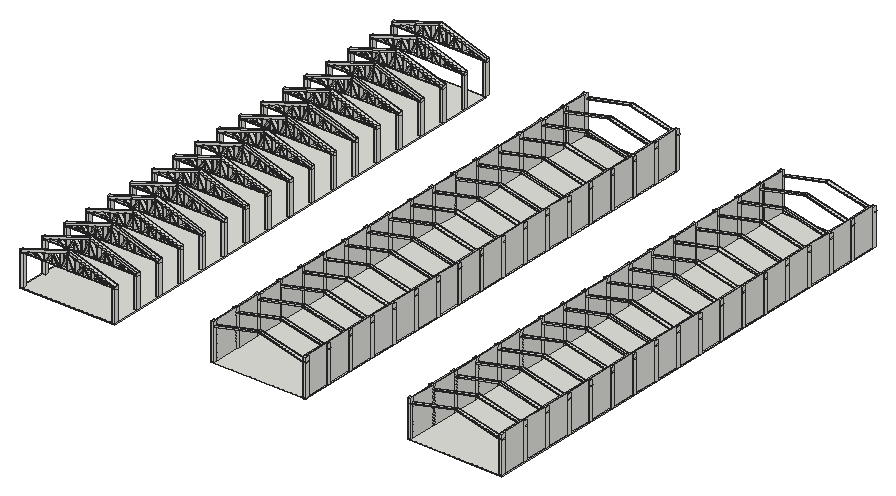
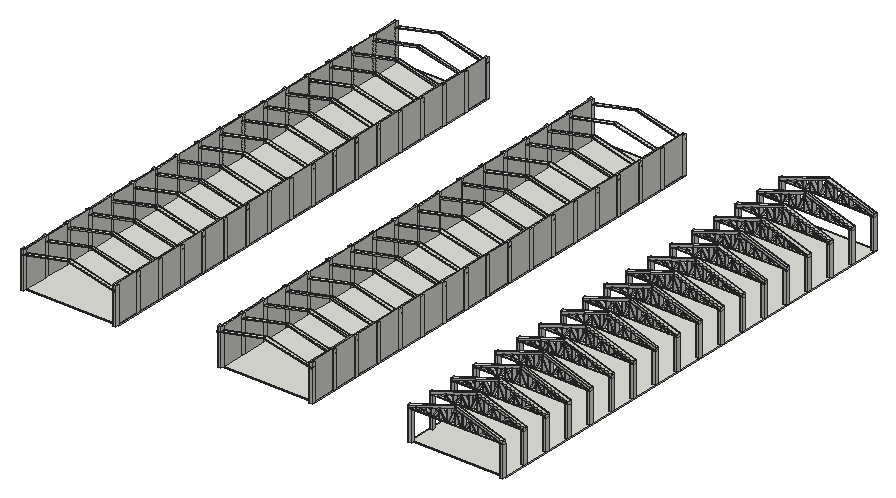
# SketchUp Ruby script. Lengths in inches.
U = 1.inch
M = Sketchup.active_model
def pt(a) = Geom::Point3d.new(a.map { |v| v * U })
def face(e, loops, mat)
  f = e.add_face(loops[0].map { |a| pt(a) })
  loops[1..].each { |l| e.add_face(l.map { |a| pt(a) }).erase! }
  f.material = f.back_material = mat if mat
  f
end
# faces: each face lists its corners as indices into pts; further lists are holes
def faces(e, pts, list, mat = nil) = list.each { |f| face(e, (f[0].is_a?(Array) ? f : [f]).map { |l| l.map { |i| pts[i] } }, mat) }
# xy, xz, yz: faces in a plane at the given z, y or x. An outline is a flat list of corners, or four numbers for a rectangle; further outlines are holes
def ring(l) = l.size == 4 ? [[l[0], l[1]], [l[2], l[1]], [l[2], l[3]], [l[0], l[3]]] : l.each_slice(2).to_a
def flat(e, list, mat, &to3) = list.each { |f| face(e, (f[0].is_a?(Array) ? f : [f]).map { |l| ring(l).map { |u, v| to3.(u, v) } }, mat) }
def xy(e, z, list, mat = nil) = flat(e, list, mat) { |x, y| [x, y, z] }
def xz(e, y, list, mat = nil) = flat(e, list, mat) { |x, z| [x, y, z] }
def yz(e, x, list, mat = nil) = flat(e, list, mat) { |y, z| [x, y, z] }
def lines(e, pts, list) = list.each { |a, b| e.add_line(pt(pts[a]), pt(pts[b])) }
# prism: a flat outline (further loops are holes) pulled along v
def prism(e, loops, v, mat = nil)
  f = face(e, loops, mat); d = Geom::Vector3d.new(v.map { |x| x * U })
  f.pushpull(f.normal.samedirection?(d) ? d.length : -d.length)
end
def box(e, o, s, mat = nil) = prism(e, [[o, [o[0] + s[0], o[1], o[2]], [o[0] + s[0], o[1] + s[1], o[2]], [o[0], o[1] + s[1], o[2]]]], [0, 0, s[2]], mat)
def at(x, y, z, deg = 0) = Geom::Transformation.translation(pt([x, y, z])) * Geom::Transformation.rotation(ORIGIN, Z_AXIS, deg.degrees)
def axes(o, x, y, z) = Geom::Transformation.new([*x, 0, *y, 0, *z, 0, *pt(o).to_a, 1])
def part(name) = M.definitions.add(name)
# library, detail: a bought-in or finely detailed component or shape, given as its bounding box
def library(name, o, s) = part(name).tap { |d| box(d.entities, o, s) }
def detail(e, o, s) = box(e.add_group.entities, o, s)
def put(e, d, t, mat = nil) = e.add_instance(d, t).tap { |i| i.material = mat if mat }
def group(e, t, mat = nil) = e.add_group.tap { |g| g.transformation = t; g.material = mat if mat }.entities
root = M.entities
c1 = part("Group\#1")
box(c1.entities,[0,0,0],[528,2580,4])
c2 = part("Group\#7")
box(c2.entities,[0,1824,0],[18,18,168])
box(c2.entities,[0,1672,0],[18,18,168])
box(c2.entities,[0,1216,0],[18,18,168])
box(c2.entities,[0,1064,0],[18,18,168])
box(c2.entities,[0,1368,0],[18,18,168])
box(c2.entities,[0,912,0],[18,18,168])
box(c2.entities,[0,1520,0],[18,18,168])
box(c2.entities,[0,152,0],[18,18,168])
box(c2.entities,[0,304,0],[18,18,168])
box(c2.entities,[0,608,0],[18,18,168])
box(c2.entities,[0,760,0],[18,18,168])
box(c2.entities,[0,0,0],[18,18,168])
box(c2.entities,[0,456,0],[18,18,168])
box(c2.entities,[0,1976,0],[18,18,168])
box(c2.entities,[0,2580,0],[18,18,168])
box(c2.entities,[0,2280,0],[18,18,168])
box(c2.entities,[0,2128,0],[18,18,168])
box(c2.entities,[0,2432,0],[18,18,168])
c3 = part("Group\#3")
box(c3.entities,[0,1824,0],[18,18,204])
box(c3.entities,[0,1672,0],[18,18,204])
box(c3.entities,[0,1216,0],[18,18,204])
box(c3.entities,[0,1064,0],[18,18,204])
box(c3.entities,[0,1368,0],[18,18,204])
box(c3.entities,[0,912,0],[18,18,204])
box(c3.entities,[0,1520,0],[18,18,204])
box(c3.entities,[0,152,0],[18,18,204])
box(c3.entities,[0,304,0],[18,18,204])
box(c3.entities,[0,608,0],[18,18,204])
box(c3.entities,[0,760,0],[18,18,204])
box(c3.entities,[0,0,0],[18,18,204])
box(c3.entities,[0,456,0],[18,18,204])
box(c3.entities,[0,1976,0],[18,18,204])
box(c3.entities,[0,2580,0],[18,18,204])
box(c3.entities,[0,2280,0],[18,18,204])
box(c3.entities,[0,2128,0],[18,18,204])
box(c3.entities,[0,2432,0],[18,18,204])
c4 = part("Group\#2")
box(c4.entities,[0,1824,0],[18,18,204])
box(c4.entities,[0,1672,0],[18,18,204])
box(c4.entities,[0,1216,0],[18,18,204])
box(c4.entities,[0,1064,0],[18,18,204])
box(c4.entities,[0,1368,0],[18,18,204])
box(c4.entities,[0,912,0],[18,18,204])
box(c4.entities,[0,1520,0],[18,18,204])
box(c4.entities,[0,152,0],[18,18,204])
box(c4.entities,[0,304,0],[18,18,204])
box(c4.entities,[0,608,0],[18,18,204])
box(c4.entities,[0,760,0],[18,18,204])
box(c4.entities,[0,0,0],[18,18,204])
box(c4.entities,[0,456,0],[18,18,204])
box(c4.entities,[0,1976,0],[18,18,204])
box(c4.entities,[0,2580,0],[18,18,204])
box(c4.entities,[0,2280,0],[18,18,204])
box(c4.entities,[0,2128,0],[18,18,204])
box(c4.entities,[0,2432,0],[18,18,204])
c5 = part("Group\#11")
box(c5.entities,[0,152,0],[10,134,204])
box(c5.entities,[0,1216,0],[10,134,204])
box(c5.entities,[0,1368,0],[10,134,204])
box(c5.entities,[0,608,0],[10,134,204])
box(c5.entities,[0,1976,0],[10,134,204])
box(c5.entities,[0,304,0],[10,134,204])
box(c5.entities,[0,1672,0],[10,134,204])
prism(c5.entities,[[[0,2562,0],[10,2562,0],[10,2432,0],[18,2432,0],[0,2428,0]]],[0,0,204])
box(c5.entities,[0,2280,0],[10,134,204])
box(c5.entities,[0,912,0],[10,134,204])
box(c5.entities,[0,1520,0],[10,134,204])
box(c5.entities,[0,2128,0],[10,134,204])
box(c5.entities,[0,456,0],[10,134,204])
box(c5.entities,[0,1064,0],[10,134,204])
box(c5.entities,[0,1824,0],[10,134,204])
box(c5.entities,[0,760,0],[10,134,204])
box(c5.entities,[0,0,0],[10,134,204])
c6 = part("Group\#6")
xz(c6.entities,0,[[3.64,6.56,264,89.41,260.36,90.56,264,102,0,18],[524.36,6.56,528,18,264,102,267.64,90.56,264,89.41],[264,89.41,267.64,90.56,264,102,260.36,90.56]])
xz(c6.entities,18,[[3.64,6.56,0,18,264,102,260.36,90.56,264,89.41],[524.36,6.56,264,89.41,267.64,90.56,264,102,528,18],[264,89.41,267.64,90.56,264,102,260.36,90.56]])
yz(c6.entities,0,[[0,0,18,18]])
yz(c6.entities,528,[[0,0,18,18]])
p = [[0,18,18],[0,0,18],[3.64,0,6.56],[3.64,18,6.56],[264,18,89.41],[267.64,18,90.56],
  [267.64,0,90.56],[264,0,89.41],[524.36,18,6.56],[524.36,0,6.56],[260.36,0,90.56],[260.36,18,90.56],
  [528,0,18],[528,18,18],[264,0,102],[264,18,102]]
faces(c6.entities,p,[[0,1,2,3],[3,4,5,6,7,2],[4,8,9,7,10,11],[12,13,8,9],[0,1,14,15],[15,14,12,13],[15,14,10,11],[14,15,5,6]])
c7 = part("Group\#4")
xy(c7.entities,4.625,[[3.64,0,524.36,18]])
xy(c7.entities,6.56,[[3.64,0,44.03,18],[44.03,0,50.03,18],[50.03,0,60.37,18],[60.37,0,87.43,18],[87.43,0,93.43,18],
  [93.43,0,120.9375,18],[120.9375,0,130.82,18],[130.82,0,136.82,18],[136.82,0,144.11,18],[144.11,0,174.21,18],
  [174.21,0,180.21,18],[180.21,0,210.4,18],[210.4,0,217.61,18],[217.61,0,223.61,18],[223.61,0,230.1875,18],
  [230.1875,0,261,18],[261,0,267,18],[267,0,297.8,18],[297.8,0,304.39,18],[304.39,0,310.39,18],
  [310.39,0,317.6,18],[317.6,0,347.79,18],[347.79,0,353.79,18],[353.79,0,383.89,18],[383.89,0,391.18,18],
  [391.18,0,397.18,18],[397.18,0,407.0625,18],[407.0625,0,434.57,18],[434.57,0,440.57,18],[440.57,0,467.63,18],
  [467.63,0,477.97,18],[477.97,0,483.97,18],[483.97,0,524.36,18]])
xy(c7.entities,89.41,[[261,0,267,18]])
xz(c7.entities,0,[[3.64,4.625,524.36,6.56],[44.03,6.56,50.03,6.56,50.03,21.33,44.03,19.42],[50.03,6.56,60.37,6.56,87.43,25.86,87.43,6.56,93.43,6.56,93.43,27.58,120.9375,6.56,130.82,6.56,93.43,35.13,87.43,33.22],[130.82,6.56,136.82,6.56,136.82,48.94,130.82,47.03],[136.82,6.56,144.11,6.56,174.21,50.26,174.21,6.56,180.21,6.56,180.21,51.92,210.4,6.56,217.61,6.56,180.21,62.75,174.21,60.84],
  [217.61,6.56,223.61,6.56,223.61,76.55,217.61,74.65],[223.61,6.56,230.1875,6.56,261,74.82,261,6.56,267,6.56,267,74.01,297.8,6.56,304.39,6.56,267,88.45,267,89.41,261,89.41],[304.39,6.56,310.39,6.56,310.39,74.65,304.39,76.55],[310.39,6.56,317.6,6.56,347.79,51.92,347.79,6.56,353.79,6.56,353.79,50.78,383.89,6.56,391.18,6.56,353.79,60.84,347.79,62.75],[391.18,6.56,397.18,6.56,397.18,47.03,391.18,48.94],
  [397.18,6.56,407.0625,6.56,434.57,27.58,434.57,6.56,440.57,6.56,440.57,25.86,467.63,6.56,477.97,6.56,440.57,33.22,440.29,33.3125,434.57,35.13],[477.97,6.56,483.97,6.56,483.97,19.42,477.97,21.33]])
xz(c7.entities,18,[[3.64,4.625,524.36,6.56],[44.03,6.56,44.03,19.42,50.03,21.33,50.03,6.56],[50.03,6.56,87.43,33.22,93.43,35.13,130.82,6.56,120.9375,6.56,93.43,27.58,93.43,6.56,87.43,6.56,87.43,25.86,60.37,6.56],[130.82,6.56,130.82,47.03,136.82,48.94,136.82,6.56],[136.82,6.56,174.21,60.84,180.21,62.75,217.61,6.56,210.4,6.56,180.21,51.92,180.21,6.56,174.21,6.56,174.21,50.26,144.11,6.56],
  [217.61,6.56,217.61,74.65,223.61,76.55,223.61,6.56],[223.61,6.56,261,89.41,267,89.41,267,88.45,304.39,6.56,297.8,6.56,267,74.01,267,6.56,261,6.56,261,74.82,230.1875,6.56],[304.39,6.56,304.39,76.55,310.39,74.65,310.39,6.56],[310.39,6.56,347.79,62.75,353.79,60.84,391.18,6.56,383.89,6.56,353.79,50.78,353.79,6.56,347.79,6.56,347.79,51.92,317.6,6.56],[391.18,6.56,391.18,48.94,397.18,47.03,397.18,6.56],
  [397.18,6.56,434.57,35.13,440.29,33.3125,440.57,33.22,477.97,6.56,467.63,6.56,440.57,25.86,440.57,6.56,434.57,6.56,434.57,27.58,407.0625,6.56],[477.97,6.56,477.97,21.33,483.97,19.42,483.97,6.56]])
yz(c7.entities,3.64,[[0,4.625,18,6.56]])
yz(c7.entities,44.03,[[0,6.56,18,19.42]])
yz(c7.entities,50.03,[[0,6.56,18,21.33]])
yz(c7.entities,87.43,[[0,6.56,18,25.86]])
yz(c7.entities,93.43,[[0,6.56,18,27.58]])
yz(c7.entities,130.82,[[0,6.56,18,47.03]])
yz(c7.entities,136.82,[[0,6.56,18,48.94]])
yz(c7.entities,174.21,[[0,6.56,18,50.26]])
yz(c7.entities,180.21,[[0,6.56,18,51.92]])
yz(c7.entities,217.61,[[0,6.56,18,74.65]])
yz(c7.entities,223.61,[[0,6.56,18,76.55]])
yz(c7.entities,261,[[0,6.56,18,74.82]])
yz(c7.entities,267,[[0,6.56,18,74.01],[0,88.45,18,89.41]])
yz(c7.entities,304.39,[[0,6.56,18,76.55]])
yz(c7.entities,310.39,[[0,6.56,18,74.65]])
yz(c7.entities,347.79,[[0,6.56,18,51.92]])
yz(c7.entities,353.79,[[0,6.56,18,50.78]])
yz(c7.entities,391.18,[[0,6.56,18,48.94]])
yz(c7.entities,397.18,[[0,6.56,18,47.03]])
yz(c7.entities,434.57,[[0,6.56,18,27.58]])
yz(c7.entities,440.57,[[0,6.56,18,25.86]])
yz(c7.entities,477.97,[[0,6.56,18,21.33]])
yz(c7.entities,483.97,[[0,6.56,18,19.42]])
yz(c7.entities,524.36,[[0,4.625,18,6.56]])
p = [[50.03,0,6.56],[87.43,0,33.22],[87.43,18,33.22],[50.03,18,6.56],[87.43,0,25.86],[60.37,0,6.56],
  [60.37,18,6.56],[87.43,18,25.86],[93.43,0,35.13],[130.82,0,6.56],[130.82,18,6.56],[93.43,18,35.13],
  [120.9375,0,6.56],[93.43,0,27.58],[93.43,18,27.58],[120.9375,18,6.56],[136.82,0,6.56],[174.21,0,60.84],
  [174.21,18,60.84],[136.82,18,6.56],[174.21,0,50.26],[144.11,0,6.56],[144.11,18,6.56],[174.21,18,50.26],
  [210.4,0,6.56],[180.21,0,51.92],[180.21,18,51.92],[210.4,18,6.56],[180.21,0,62.75],[217.61,0,6.56],
  [217.61,18,6.56],[180.21,18,62.75],[223.61,0,6.56],[261,0,89.41],[261,18,89.41],[223.61,18,6.56],
  [261,0,74.82],[230.1875,0,6.56],[230.1875,18,6.56],[261,18,74.82],[297.8,0,6.56],[267,0,74.01],
  [267,18,74.01],[297.8,18,6.56],[267,0,88.45],[304.39,0,6.56],[304.39,18,6.56],[267,18,88.45],
  [310.39,0,6.56],[347.79,0,62.75],[347.79,18,62.75],[310.39,18,6.56],[347.79,0,51.92],[317.6,0,6.56],
  [317.6,18,6.56],[347.79,18,51.92],[383.89,0,6.56],[353.79,0,50.78],[353.79,18,50.78],[383.89,18,6.56],
  [353.79,0,60.84],[391.18,0,6.56],[391.18,18,6.56],[353.79,18,60.84],[397.18,0,6.56],[434.57,0,35.13],
  [434.57,18,35.13],[397.18,18,6.56],[434.57,0,27.58],[407.0625,0,6.56],[407.0625,18,6.56],[434.57,18,27.58],
  [440.57,0,33.22],[477.97,0,6.56],[477.97,18,6.56],[440.57,18,33.22],[467.63,0,6.56],[440.57,0,25.86],
  [440.57,18,25.86],[467.63,18,6.56],[44.03,0,19.42],[50.03,0,21.33],[50.03,18,21.33],[44.03,18,19.42],
  [477.97,0,21.33],[483.97,0,19.42],[483.97,18,19.42],[477.97,18,21.33],[440.29,0,33.3125],[440.29,18,33.3125],
  [130.82,0,47.03],[136.82,0,48.94],[136.82,18,48.94],[130.82,18,47.03],[391.18,0,48.94],[397.18,0,47.03],
  [397.18,18,47.03],[391.18,18,48.94],[217.61,0,74.65],[223.61,0,76.55],[223.61,18,76.55],[217.61,18,74.65],
  [304.39,0,76.55],[310.39,0,74.65],[310.39,18,74.65],[304.39,18,76.55],[3.64,0,4.625],[0,0,0]]
faces(c7.entities,p,[[0,1,2,3],[4,5,6,7],[8,9,10,11],[12,13,14,15],[16,17,18,19],[20,21,22,23],[24,25,26,27],[28,29,30,31],
  [32,33,34,35],[36,37,38,39],[40,41,42,43],[44,45,46,47],[48,49,50,51],[52,53,54,55],[56,57,58,59],[60,61,62,63],
  [64,65,66,67],[68,69,70,71],[72,73,74,75],[76,77,78,79],[80,81,82,83],[84,85,86,87],[1,8,11,2],[88,72,75,89],
  [65,88,89,66],[90,91,92,93],[94,95,96,97],[17,28,31,18],[49,60,63,50],[98,99,100,101],[102,103,104,105]])
lines(c7.entities,p,[[106,107],[91,17],[28,98],[8,90],[81,1]])
c8 = part("Group\#8")
xz(c8.entities,0,[[1.33,0,264,59.7,262.67,60,264,65.85,0,5.85],[526.67,0,528,5.85,264,65.85,265.33,60,264,59.7],[264,59.7,262.67,60,264,65.85,265.33,60]])
xz(c8.entities,18,[[1.33,0,0,5.85,264,65.85,262.67,60,264,59.7],[526.67,0,528,5.85,264,65.85,265.33,60,264,59.7],[264,59.7,265.33,60,264,65.85,262.67,60]])
p = [[0,0,5.85],[0,18,5.85],[1.33,18,0],[1.33,0,0],[264,18,59.7],[265.33,18,60],
  [265.33,0,60],[264,0,59.7],[526.67,18,0],[262.67,18,60],[262.67,0,60],[526.67,0,0],
  [528,0,5.85],[528,18,5.85],[264,0,65.85],[264,18,65.85]]
faces(c8.entities,p,[[0,1,2,3],[3,2,4,5,6,7],[8,4,9,10,7,11],[12,13,8,11],[1,0,14,15],[14,12,13,15],[15,14,10,9],[15,14,6,5]])
put(root,c1,at(1.82,0,0))
put(root,c1,at(1062.94,0,0))
put(root,c1,at(2157.26,0,0))
put(root,c2,at(1.82,0,4))
put(root,c2,at(511.82,0,4))
put(root,c3,at(1062.94,0,4))
put(root,c4,at(1572.94,0,4))
put(root,c5,at(1572.94,18,4))
put(root,c5,at(1070.94,18,4))
put(root,c5,at(2667.26,18,4))
put(root,c5,at(2165.26,18,4))
put(root,c4,at(2667.26,0,4))
put(root,c3,at(2157.26,0,4))
put(root,c6,at(1.82,0,172))
put(root,c7,at(1.82,0,172))
put(root,c7,at(1.82,152,172))
put(root,c6,at(1.82,152,172))
put(root,c6,at(1.82,304,172))
put(root,c7,at(1.82,304,172))
put(root,c7,at(1.82,456,172))
put(root,c6,at(1.82,456,172))
put(root,c6,at(1.82,608,172))
put(root,c7,at(1.82,608,172))
put(root,c6,at(1.82,760,172))
put(root,c7,at(1.82,760,172))
put(root,c6,at(1.82,912,172))
put(root,c7,at(1.82,912,172))
put(root,c7,at(1.82,1064,172))
put(root,c6,at(1.82,1064,172))
put(root,c6,at(1.82,1216,172))
put(root,c7,at(1.82,1216,172))
put(root,c6,at(1.82,1368,172))
put(root,c7,at(1.82,1368,172))
put(root,c7,at(1.82,1520,172))
put(root,c6,at(1.82,1520,172))
put(root,c6,at(1.82,1672,172))
put(root,c7,at(1.82,1672,172))
put(root,c6,at(1.82,1824,172))
put(root,c7,at(1.82,1824,172))
put(root,c6,at(1.82,1976,172))
put(root,c7,at(1.82,1976,172))
put(root,c7,at(1.82,2128,172))
put(root,c6,at(1.82,2128,172))
put(root,c7,at(1.82,2280,172))
put(root,c6,at(1.82,2280,172))
put(root,c6,at(1.82,2432,172))
put(root,c7,at(1.82,2432,172))
put(root,c7,at(1.82,2584,172))
put(root,c6,at(1.82,2584,172))
put(root,c8,at(1063.88,0,178.17))
put(root,c8,at(1063.88,152,178.17))
put(root,c8,at(1063.88,304,178.17))
put(root,c8,at(1063.88,456,178.17))
put(root,c8,at(1063.88,608,178.17))
put(root,c8,at(1063.88,760,178.17))
put(root,c8,at(1063.88,912,178.17))
put(root,c8,at(1063.88,1064,178.17))
put(root,c8,at(1063.88,1216,178.17))
put(root,c8,at(1063.88,1368,178.17))
put(root,c8,at(1063.88,1520,178.17))
put(root,c8,at(1063.88,1672,178.17))
put(root,c8,at(1063.88,1824,178.17))
put(root,c8,at(1063.88,1976,178.17))
put(root,c8,at(1063.88,2128,178.17))
put(root,c8,at(1063.88,2280,178.17))
put(root,c8,at(1063.88,2432,178.17))
put(root,c8,at(1063.88,2584,178.17))
put(root,c8,at(2158.19,1672,178.17))
put(root,c8,at(2158.19,304,178.17))
put(root,c8,at(2158.19,2280,178.17))
put(root,c8,at(2158.19,1520,178.17))
put(root,c8,at(2158.19,1216,178.17))
put(root,c8,at(2158.19,1368,178.17))
put(root,c8,at(2158.19,2432,178.17))
put(root,c8,at(2158.19,608,178.17))
put(root,c8,at(2158.19,152,178.17))
put(root,c8,at(2158.19,2584,178.17))
put(root,c8,at(2158.19,912,178.17))
put(root,c8,at(2158.19,456,178.17))
put(root,c8,at(2158.19,2128,178.17))
put(root,c8,at(2158.19,1064,178.17))
put(root,c8,at(2158.19,760,178.17))
put(root,c8,at(2158.19,1976,178.17))
put(root,c8,at(2158.19,0,178.17))
put(root,c8,at(2158.19,1824,178.17))
